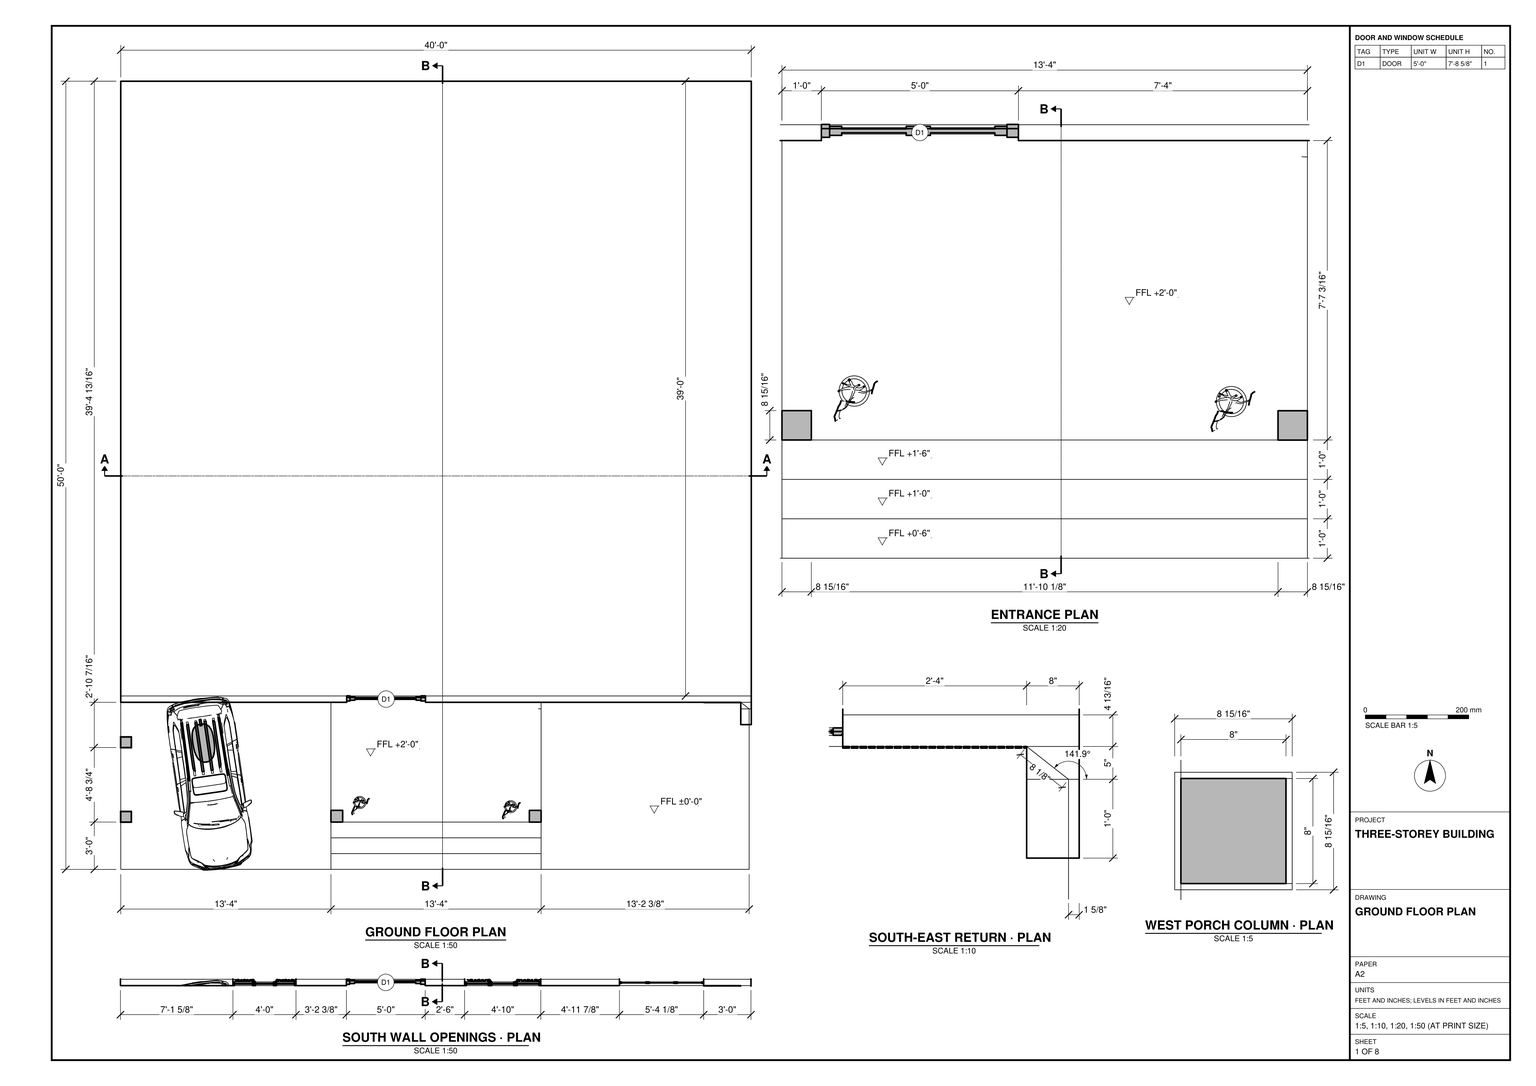
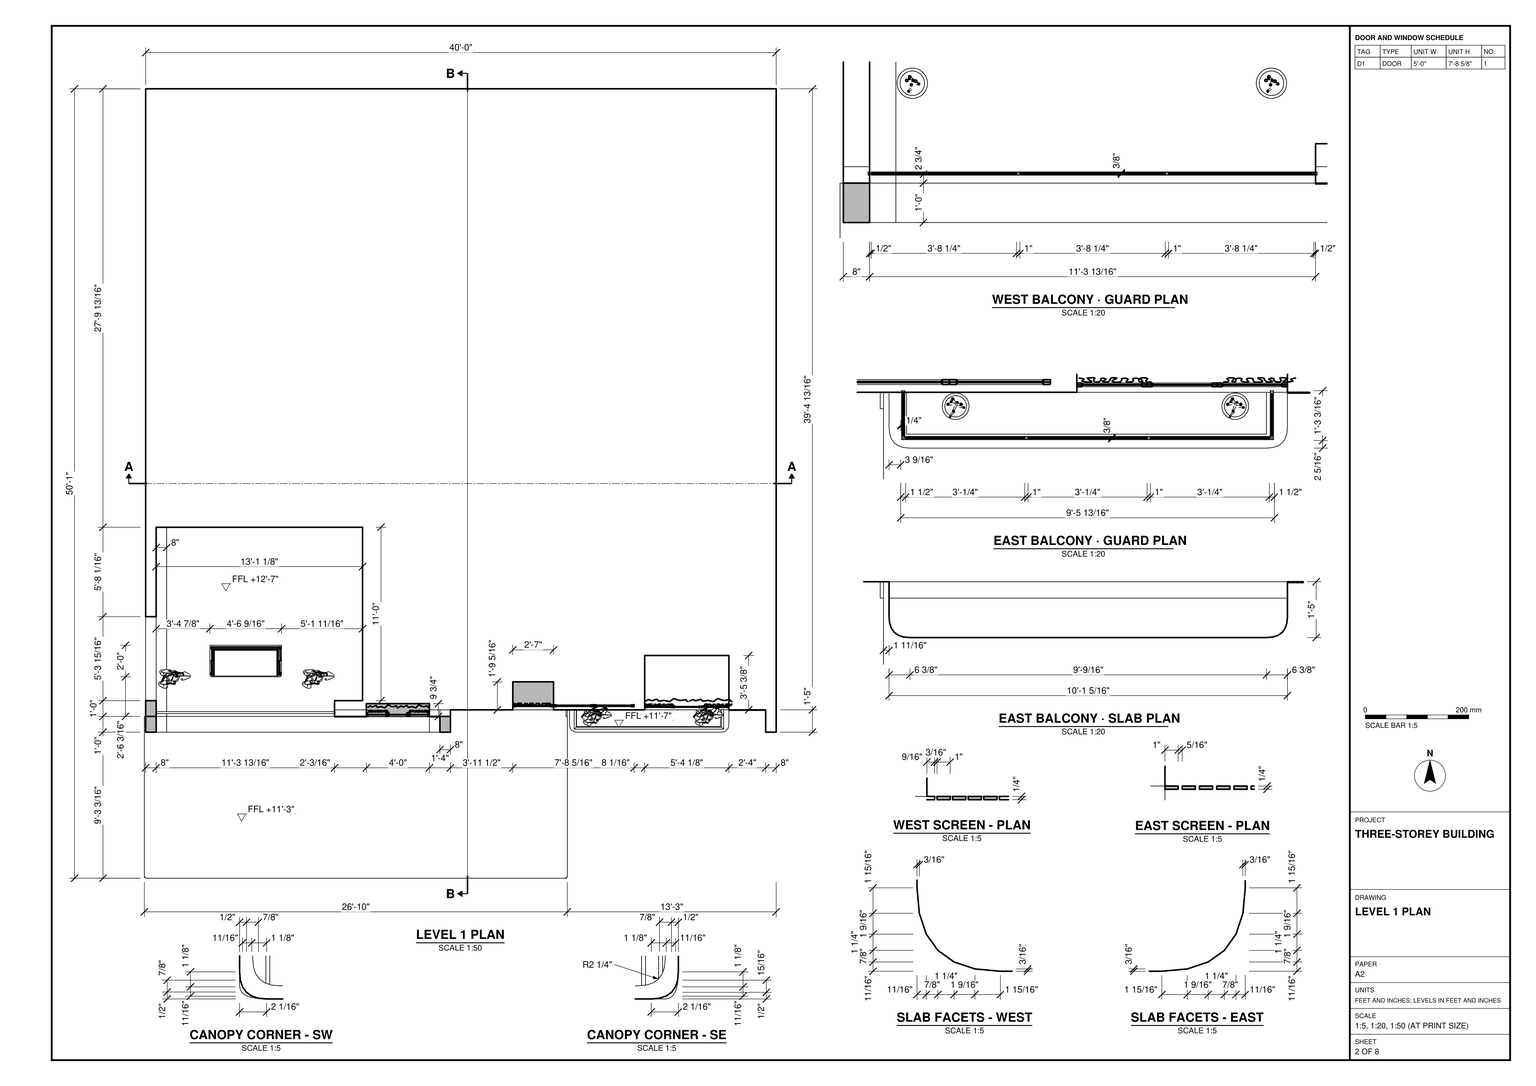
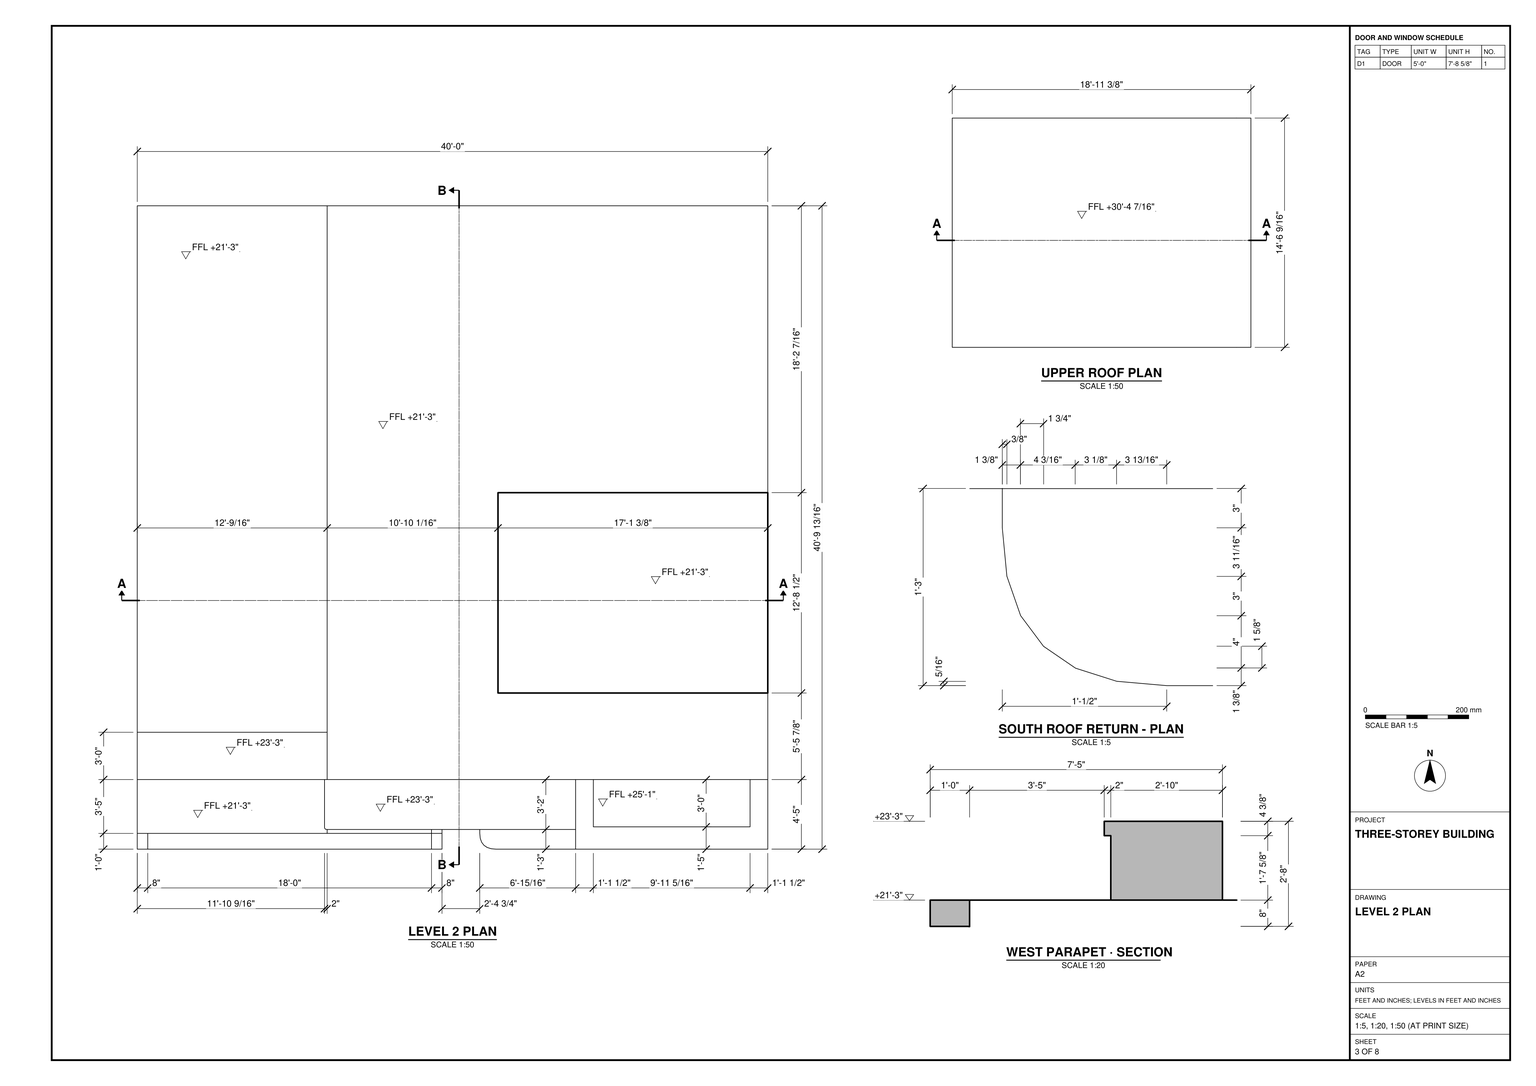
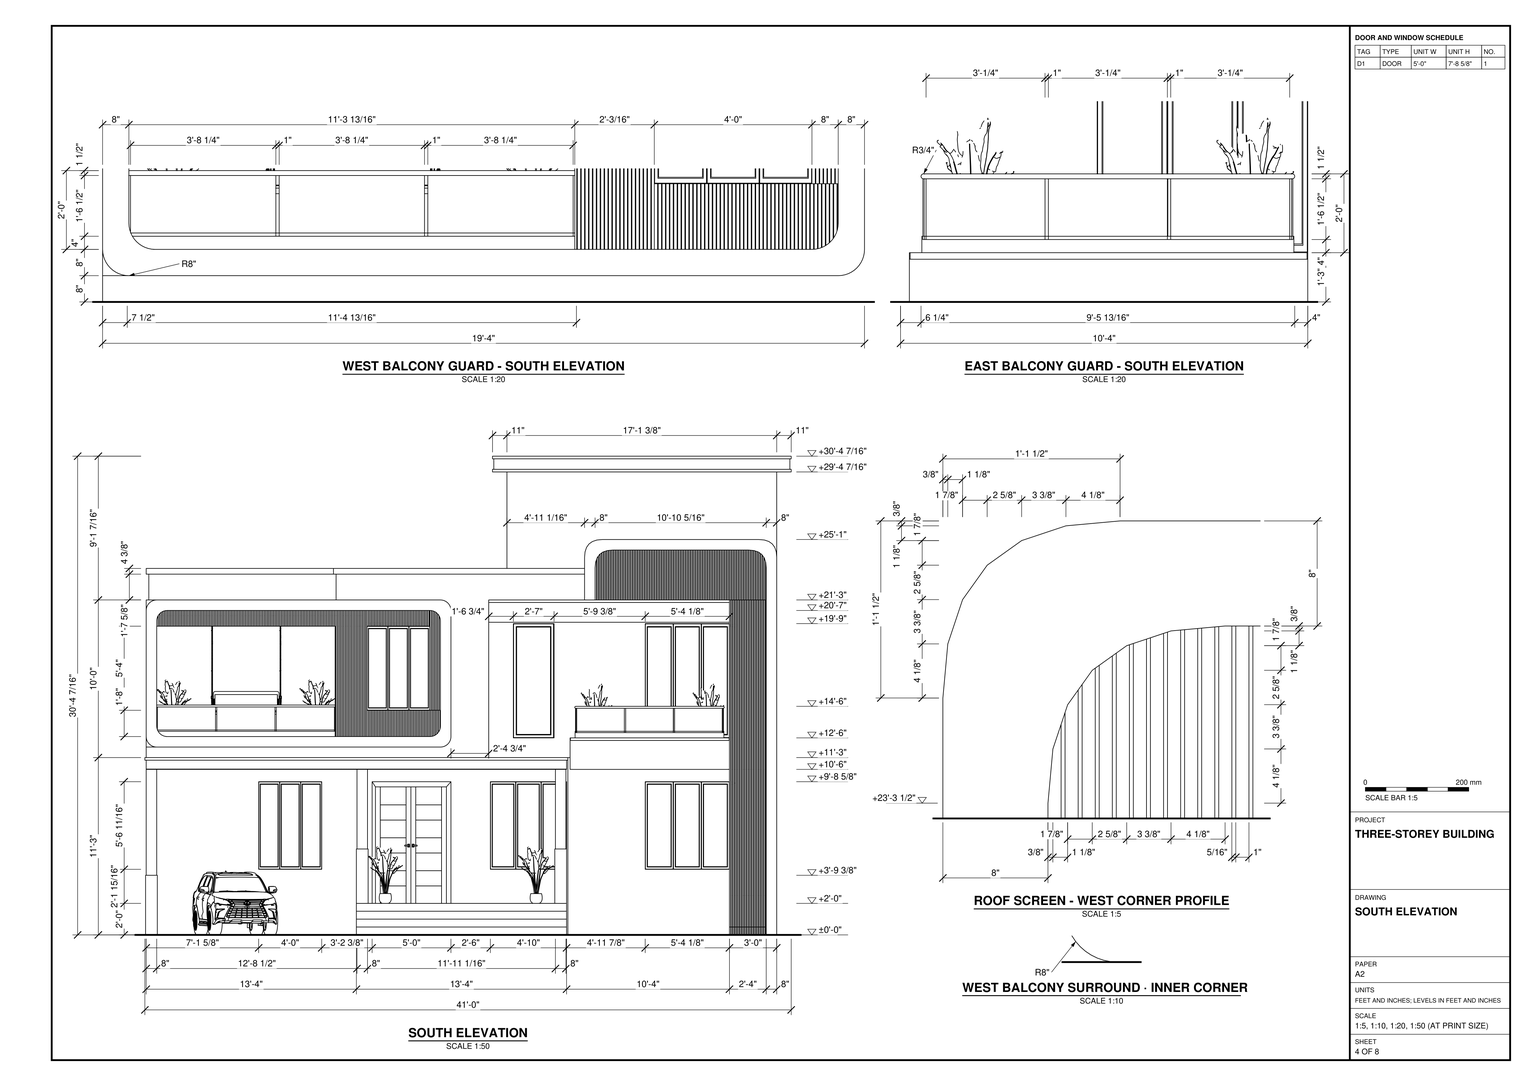
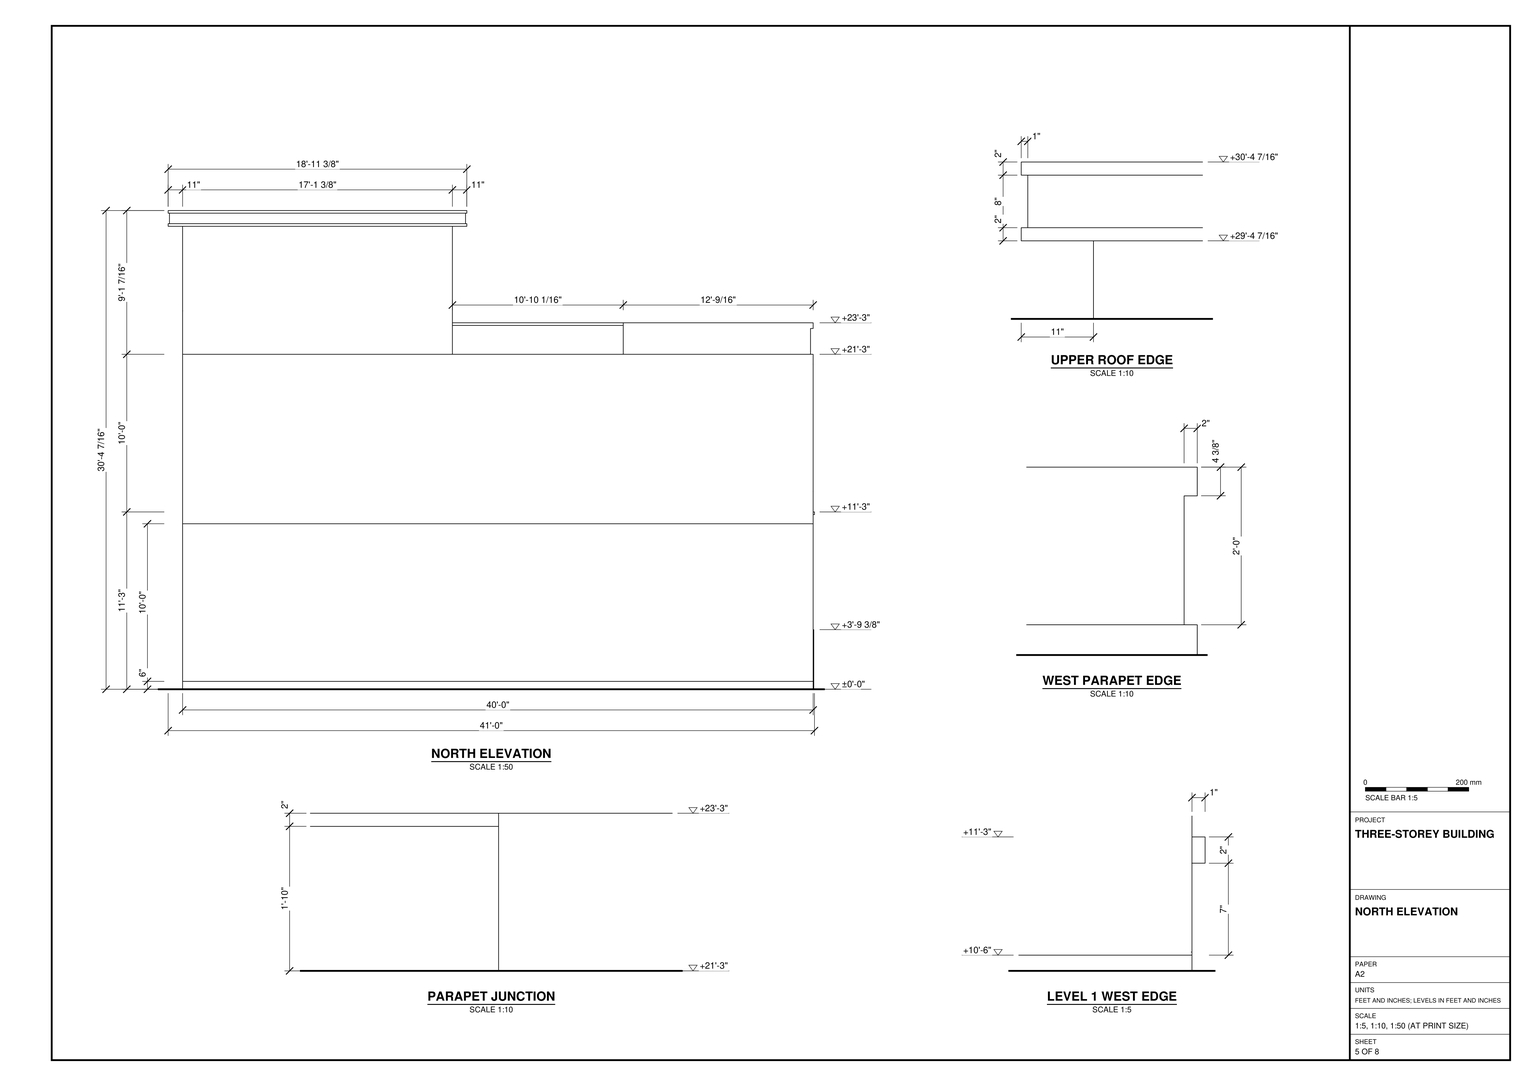
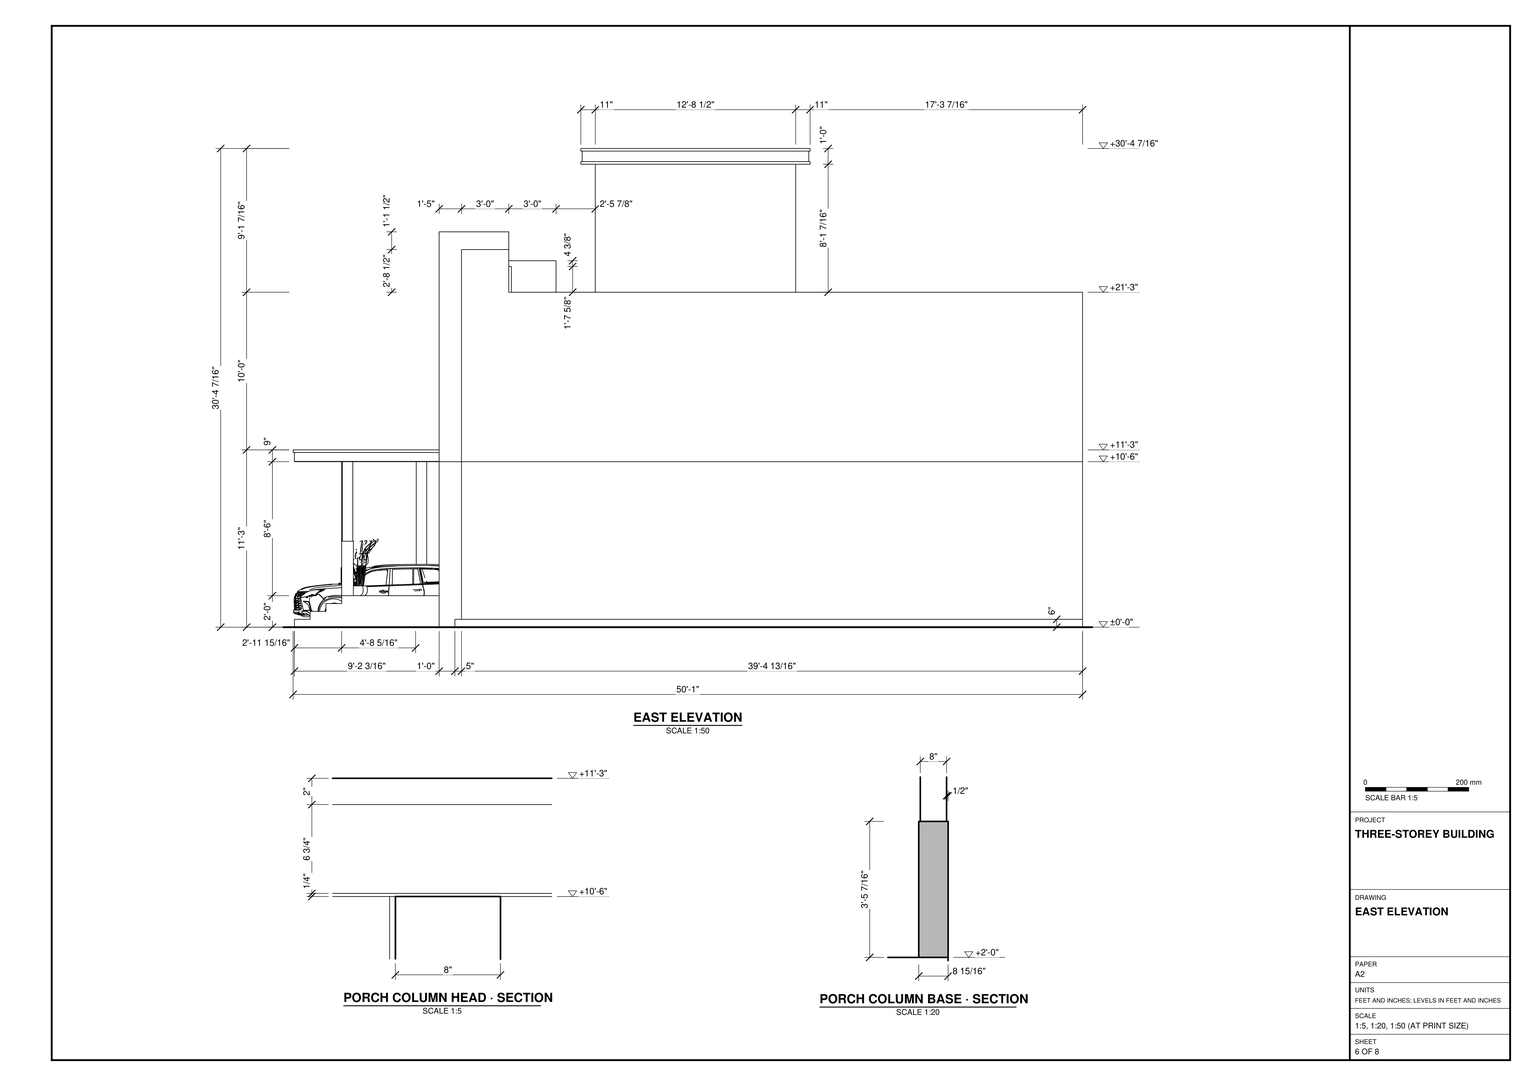
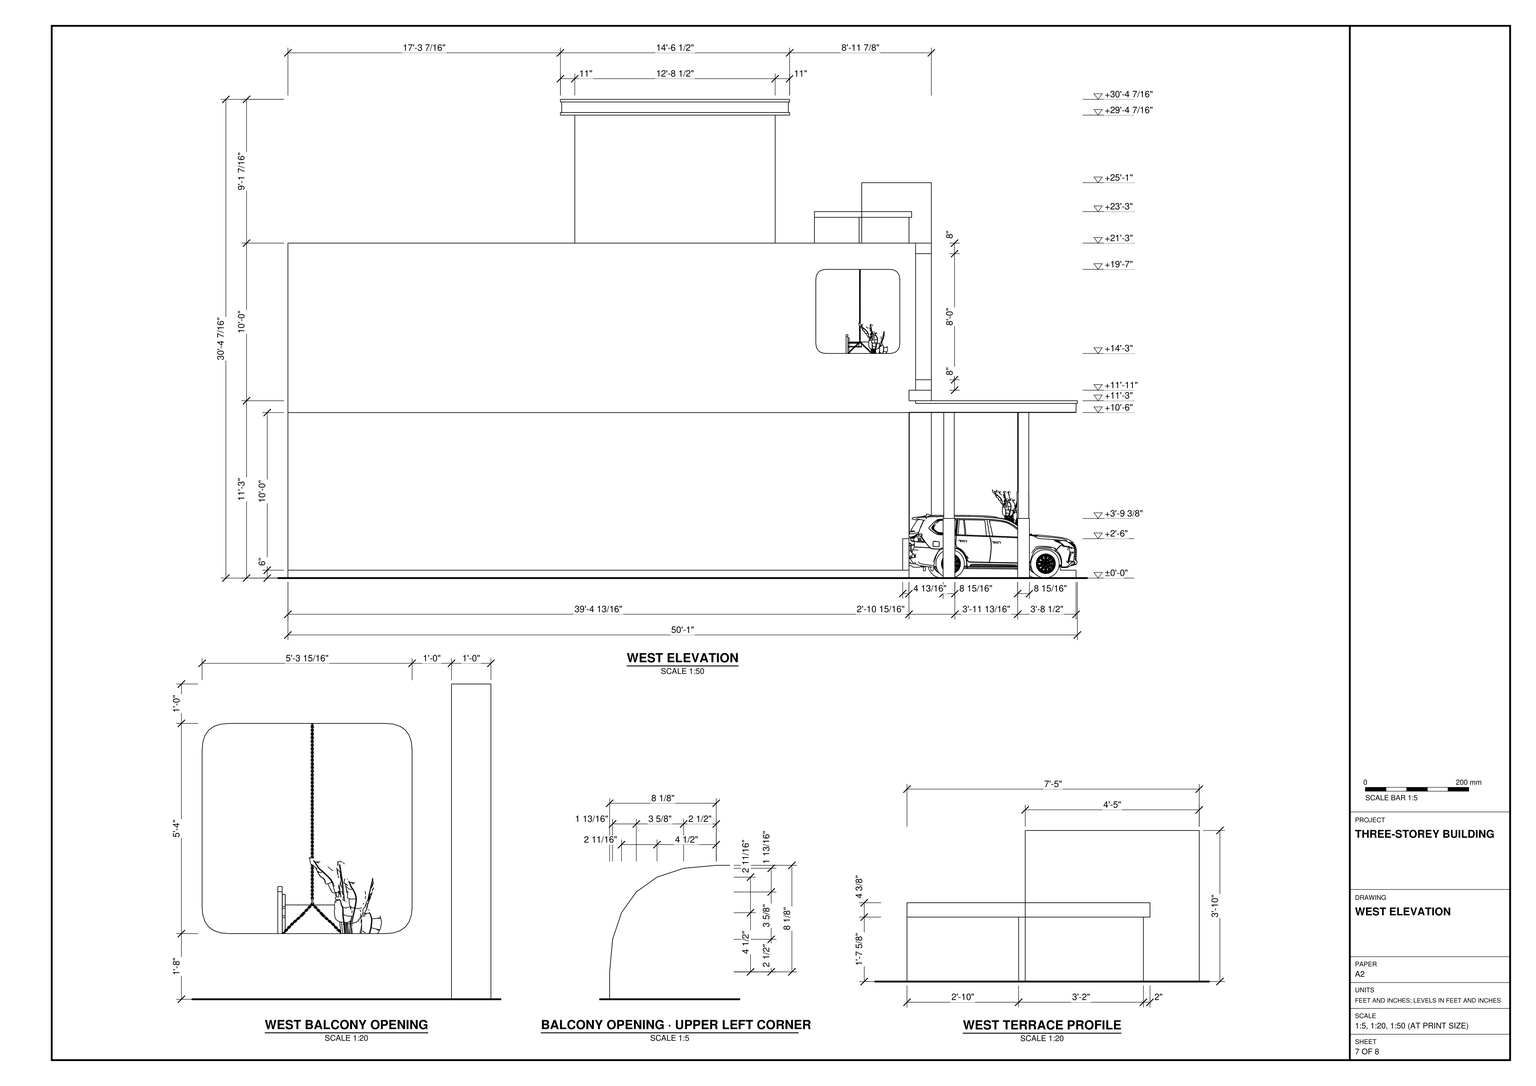
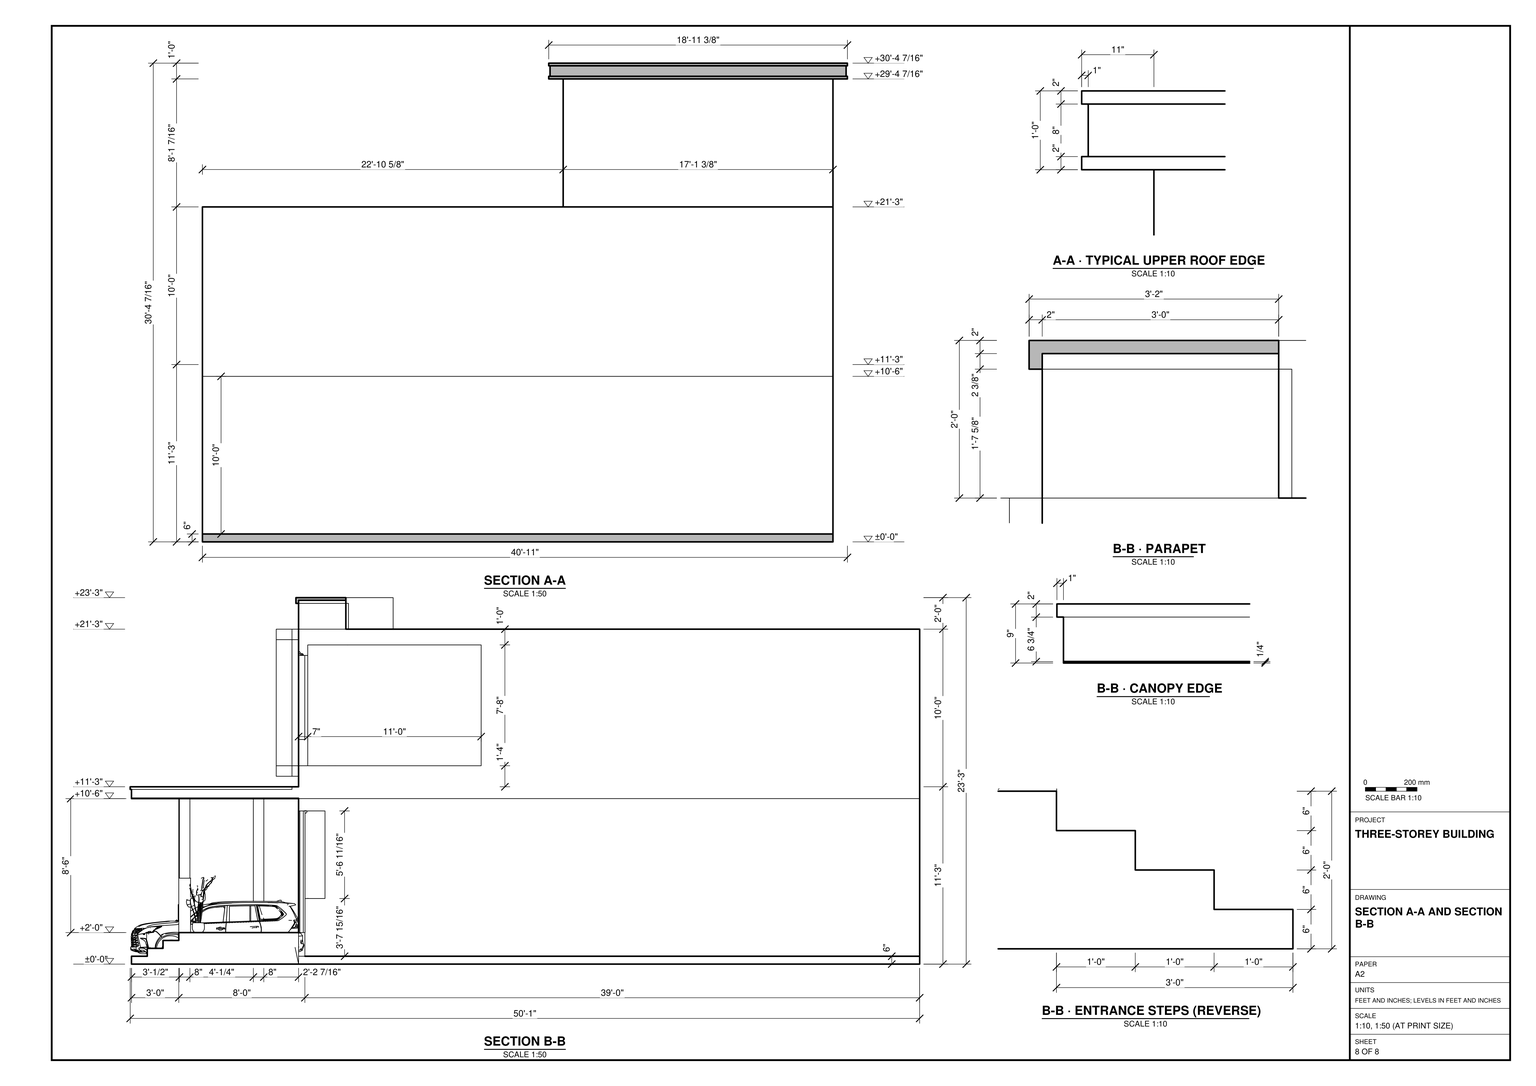
Build the three-storey building in SketchUp from task_files/diagram_01.pdf. Work in feet and inches. The overall model measures 41'-0" along X, 50'-1" along Y and 30'-4 7/16" along Z. Set the ground floor at ±0'-0", Level 1 at +11'-3" and Level 2 at +21'-3". Use the local levels on the sheets for the entrance landing, balconies and parapets.

Lay out the south frontage with the parking bay on the west and the stepped entrance in the middle bay. Carry the steps across the landing frontage and place the double door at the offset shown in the entrance plan. Model the walls at their drawn thicknesses, including the south-east return, and follow the south wall opening layout. Form the floor slabs and the canopy over the parking bay and entrance. Distinguish the recessed west balcony with its straight glass guard from the shallow projecting east balcony with its rounded slab corners and returning guard. Include the screens, parapets, smaller upper enclosure and flat upper roof. Place the vehicle, built-in joinery and main furniture where shown. Decor and loose items may be any suitable library components.

Keep walls, slabs, roof and each furniture or joinery piece in separate groups or components, and use components for repeated parts. Save one SketchUp model as output_files/three_storey_building_with_entrance_steps_and_balconies.skp.

# SketchUp Ruby script. Lengths in inches.
U = 1.inch
M = Sketchup.active_model
def pt(a) = Geom::Point3d.new(a.map { |v| v * U })
def face(e, loops, mat)
  f = e.add_face(loops[0].map { |a| pt(a) })
  loops[1..].each { |l| e.add_face(l.map { |a| pt(a) }).erase! }
  f.material = f.back_material = mat if mat
  f
end
# faces: each face lists its corners as indices into pts; further lists are holes
def faces(e, pts, list, mat = nil) = list.each { |f| face(e, (f[0].is_a?(Array) ? f : [f]).map { |l| l.map { |i| pts[i] } }, mat) }
# xy, xz, yz: faces in a plane at the given z, y or x. An outline is a flat list of corners, or four numbers for a rectangle; further outlines are holes
def ring(l) = l.size == 4 ? [[l[0], l[1]], [l[2], l[1]], [l[2], l[3]], [l[0], l[3]]] : l.each_slice(2).to_a
def flat(e, list, mat, &to3) = list.each { |f| face(e, (f[0].is_a?(Array) ? f : [f]).map { |l| ring(l).map { |u, v| to3.(u, v) } }, mat) }
def xy(e, z, list, mat = nil) = flat(e, list, mat) { |x, y| [x, y, z] }
def xz(e, y, list, mat = nil) = flat(e, list, mat) { |x, z| [x, y, z] }
def yz(e, x, list, mat = nil) = flat(e, list, mat) { |y, z| [x, y, z] }
def lines(e, pts, list) = list.each { |a, b| e.add_line(pt(pts[a]), pt(pts[b])) }
# prism: a flat outline (further loops are holes) pulled along v
def prism(e, loops, v, mat = nil)
  f = face(e, loops, mat); d = Geom::Vector3d.new(v.map { |x| x * U })
  f.pushpull(f.normal.samedirection?(d) ? d.length : -d.length)
end
def box(e, o, s, mat = nil) = prism(e, [[o, [o[0] + s[0], o[1], o[2]], [o[0] + s[0], o[1] + s[1], o[2]], [o[0], o[1] + s[1], o[2]]]], [0, 0, s[2]], mat)
def at(x, y, z, deg = 0) = Geom::Transformation.translation(pt([x, y, z])) * Geom::Transformation.rotation(ORIGIN, Z_AXIS, deg.degrees)
def axes(o, x, y, z) = Geom::Transformation.new([*x, 0, *y, 0, *z, 0, *pt(o).to_a, 1])
def part(name) = M.definitions.add(name)
# library, detail: a bought-in or finely detailed component or shape, given as its bounding box
def library(name, o, s) = part(name).tap { |d| box(d.entities, o, s) }
def detail(e, o, s) = box(e.add_group.entities, o, s)
def put(e, d, t, mat = nil) = e.add_instance(d, t).tap { |i| i.material = mat if mat }
def group(e, t, mat = nil) = e.add_group.tap { |g| g.transformation = t; g.material = mat if mat }.entities
root = M.entities
M.materials.add("POT_TEXTURE_1").color = [172, 172, 172]
M.materials.add("[0136_Charcoal]").color = [35, 35, 35]
M.materials.add("soil1").color = [68, 55, 47]
M.materials.add("тюль").color = [255, 255, 255]
c1 = part("Group\#61")
p = [[0,1.89,0.38],[0,1.89,1.61],[0,0.72,0],[0,0,0.99],[0,0.72,1.99]]
lines(c1.entities,p,[[0,1],[2,0],[3,2],[4,3],[1,4]])
c2 = part("Pleated curtain panel")
xz(c2.entities,2.13,[[4.6,2.7,5.13,80]])
xz(c2.entities,5.27,[[15.31,2.7,16.125,80]])
yz(c2.entities,16.67,[[3.29,2.7,4.74,80]])
# 1 loose lines left out
p = [[1.66,2.25,2.7],[3.22,1.93,2.7],[3.22,1.93,80],[1.66,2.25,80],[3.53,2.38,2.7],[3.53,2.38,80],
  [9.86,2.02,2.7],[10.31,1.94,2.7],[10.31,1.94,80],[9.86,2.02,80],[11.57,2.08,2.7],[11.57,2.08,80],
  [9.23,2.61,2.7],[9.23,2.61,80],[4.47,2.21,2.7],[4.6,2.13,2.7],[4.6,2.13,80],[4.47,2.21,80],
  [5.13,2.13,2.7],[5.61,2.42,2.7],[5.61,2.42,80],[5.13,2.13,80],[11.91,3.91,2.7],[11.91,3.91,80],
  [13.07,2.39,2.7],[13.2,2.07,2.7],[13.2,2.07,80],[13.07,2.39,80],[13.86,2.05,2.7],[13.86,2.05,80],
  [14.78,2.36,2.7],[14.78,2.36,80],[19.11,2.17,2.7],[19.64,2.13,2.7],[19.64,2.13,80],[19.11,2.17,80],
  [20.05,2.2,80],[20.05,2.2,2.7],[0.73,2.89,2.7],[0.73,2.89,80],[4.17,2.57,2.7],[4.17,2.57,80],
  [6.63,2.37,2.7],[7.21,2.1875,2.7],[7.21,2.1875,80],[6.63,2.37,80],[8.1,2.21,2.7],[8.1,2.21,80],
  [8.6875,3.87,2.7],[8.6875,3.87,80],[18.86,2.29,2.7],[18.86,2.29,80],[16.86,2.42,2.7],[17.27,2.32,2.7],
  [17.27,2.32,80],[16.86,2.42,80],[17.64,2.3,2.7],[17.64,2.3,80],[17.8,2.47,2.7],[17.8,2.47,80],
  [18.73,2.57,2.7],[18.73,2.57,80],[2.85,3.77,2.7],[2.85,3.77,80],[6.16,3.6875,2.7],[6.16,3.6875,80],
  [6.49,2.63,2.7],[6.49,2.63,80],[13.52,3.66,2.7],[13.52,3.66,80],[15.24,3.3,2.7],[15.24,3.3,80],
  [16.73,2.58,2.7],[16.73,2.58,80],[17.43,3.97,2.7],[17.43,3.97,80],[3.97,3.43,2.7],[3.97,3.43,80],
  [7.51,4.62,2.7],[7.51,4.62,80],[9.28,3.38,2.7],[9.28,3.38,80],[16.67,3.29,2.7],[16.67,3.29,80],
  [18.67,3.61,2.7],[18.67,3.61,80],[0.95,3.36,2.7],[0.95,3.36,80],[14.95,4.9,2.7],[14.95,4.9,80],
  [1.38,4.43,2.7],[1.38,4.43,80],[4.41,5.3125,2.7],[4.41,5.3125,80],[10.52,5.17,2.7],[10.52,5.17,80],
  [19.17,4.87,2.7],[19.17,4.87,80],[6.02,5.06,2.7],[6.02,5.06,80],[13.64,4.74,2.7],[13.64,4.74,80],
  [2.23,5.46,2.7],[2.23,5.46,80],[8.72,5.1,2.7],[8.72,5.1,80],[11.87,5.08,2.7],[11.87,5.08,80],
  [17.03,5.16,2.7],[17.03,5.16,80],[0.95,4.94,2.7],[0.95,4.94,80],[6.82,5.39,2.7],[6.82,5.39,80],
  [13.01,5.35,2.7],[13.01,5.35,80],[16.125,5.27,2.7],[16.67,4.74,2.7],[16.67,4.74,80],[16.125,5.27,80],
  [0,5.49,2.7],[0,5.49,80],[15.31,5.27,2.7],[15.31,5.27,80],[18.65,5.66,2.7],[18.65,5.66,80],
  [9.31,5.76,2.7],[9.31,5.76,80],[10.5,5.58,2.7],[10.5,5.58,80],[17.3,5.61,80],[17.3,5.61,2.7],
  [3.98,5.8,2.7],[3.98,5.8,80]]
faces(c2.entities,p,[[0,1,2,3],[1,4,5,2],[6,7,8,9],[7,10,11,8],[12,6,9,13],[14,15,16,17],[18,19,20,21],[10,22,23,11],
  [24,25,26,27],[25,28,29,26],[28,30,31,29],[32,33,34,35],[36,34,33,37],[38,0,3,39],[40,14,17,41],[42,43,44,45],
  [43,46,47,44],[46,48,49,47],[50,32,35,51],[52,53,54,55],[53,56,57,54],[56,58,59,57],[60,50,51,61],[4,62,63,5],
  [19,64,65,20],[66,42,45,67],[68,24,27,69],[30,70,71,31],[72,52,55,73],[58,74,75,59],[76,40,41,77],[78,66,67,79],
  [80,12,13,81],[82,72,73,83],[84,60,61,85],[86,38,39,87],[70,88,89,71],[90,86,87,91],[92,76,77,93],[94,80,81,95],
  [96,84,85,97],[64,98,99,65],[100,68,69,101],[62,102,103,63],[48,104,105,49],[22,106,107,23],[74,108,109,75],[110,90,91,111],
  [112,78,79,113],[114,100,101,115],[116,117,118,119],[120,110,111,121],[88,122,123,89],[124,96,97,125],[98,112,113,99],[104,126,127,105],
  [106,114,115,107],[128,94,95,129],[130,109,108,131],[132,92,93,133],[102,132,133,103],[126,128,129,127],[131,124,125,130]])
put(c2.entities,c1,at(9.77,5.02,80,-180))
put(c2.entities,c1,at(11.91,5.02,80,-180))
put(c2.entities,c1,at(13.54,5.02,80,-180))
put(c2.entities,c1,at(7.29,5.02,80,-180))
put(c2.entities,c1,at(6.18,5.02,80,-180))
put(c2.entities,c1,at(8.69,5.02,80,-180))
put(c2.entities,c1,at(17.42,5.04,80,-180))
put(c2.entities,c1,at(18.86,5.04,80,-180))
put(c2.entities,c1,at(15.09,5.02,80,-180))
put(c2.entities,c1,at(16.66,5.04,80,-180))
put(c2.entities,c1,at(2.54,5.02,80,-180))
put(c2.entities,c1,at(1.38,5.02,80,-180))
put(c2.entities,c1,at(4.1,5.02,80,-180))
c3 = part("end")
yz(c3.entities,0,[[1.28,1.02,0.97,1.12,0.97,1.45,1.28,1.55,1.48,1.28]])
p = [[2,0,0.49],[0,0.97,1.12],[0,1.28,1.02],[2,1.51,0],[4,0.54,0.84],[4,1.38,0.57],
  [0,1.48,1.28],[2,2.44,1.28],[4,1.9,1.28],[2,0,2.08],[0,0.97,1.45],[4,0.54,1.72],
  [0,1.28,1.55],[2,1.51,2.57],[4,1.38,2]]
faces(c3.entities,p,[[0,1,2,3],[4,0,3,5],[3,2,6,7],[3,7,8,5],[0,9,10,1],[4,11,9,0],[6,12,13,7],[7,13,14,8],
  [13,12,10,9],[14,13,9,11]])
c4 = part("Component\#75")
p = [[0,2.02,1.1875],[0,1.01,1.92],[0,1.64,0],[0,0,1.1875],[0,0.39,0]]
lines(c4.entities,p,[[0,1],[2,0],[3,4],[4,2],[1,3]])
c5 = part("Shower curtain\#1")
xy(c5.entities,-0.5,[[27.83,-0.5,97.78,0]],"[0136_Charcoal]")
xy(c5.entities,0,[[27.83,-0.5,97.78,0]],"[0136_Charcoal]")
xz(c5.entities,-0.5,[[27.83,-0.5,97.78,0]],"[0136_Charcoal]")
xz(c5.entities,0,[[27.83,-0.5,97.78,0]],"[0136_Charcoal]")
yz(c5.entities,27.83,[[-0.5,-0.5,0,0]])
yz(c5.entities,97.78,[[-0.5,-0.5,0,0]],"[0136_Charcoal]")
put(c5.entities,c4,at(16.28,-1.32,-1.6875))
put(c5.entities,c4,at(12.125,-1.32,-1.6875))
put(c5.entities,c4,at(25.09,-1.32,-1.6875))
put(c5.entities,c4,at(7.66,-1.32,-1.6875))
put(c5.entities,c4,at(37.05,-1.32,-1.6875))
put(c5.entities,c4,at(48.17,-1.32,-1.6875))
put(c5.entities,c4,at(29.99,-1.32,-1.6875))
put(c5.entities,c4,at(34.45,-1.32,-1.6875))
put(c5.entities,c4,at(58.19,-1.32,-1.6875))
put(c5.entities,c4,at(52.32,-1.32,-1.6875))
put(c5.entities,c4,at(3.19,-1.32,-1.6875))
put(c5.entities,c4,at(21.06,-1.32,-1.6875))
put(c5.entities,c4,at(43.39,-1.32,-1.6875))
g1 = group(c5.entities,at(0.71,-1.3,-104.16))
p = [[26.9375,4.31,0],[20.6,5.3,0.1],[20.6,0.99,102.68],[26.9375,0,102.58],[31.63,6.62,0.24],[31.63,2.31,102.82],
  [47.72,4.31,0],[46.34,4.86,0.06],[46.34,0.55,102.64],[47.72,0,102.58],[14.89,4.64,0.03],[12.6875,6.18,0.19],
  [12.6875,1.87,102.77],[14.89,0.33,102.61],[3.59,5.85,0.16],[0,4.86,0.06],[0,0.55,102.64],[3.59,1.54,102.74],
  [45.42,5.85,0.16],[45.42,1.54,102.74],[6.9,4.97,0.07],[6.9,0.66,102.65],[39.72,5.1875,0.09],[35.58,5.625,0.14],
  [35.58,1.32,102.72],[39.72,0.88,102.67],[34.85,6.07,0.18],[34.85,1.76,102.76]]
faces(g1,p,[[0,1,2,3],[4,0,3,5],[6,7,8,9],[10,11,12,13],[1,10,13,2],[14,15,16,17],[7,18,19,8],[20,14,17,21],
  [11,20,21,12],[22,23,24,25],[18,22,25,19],[23,26,27,24],[26,4,5,27]],"тюль")
g2 = group(c5.entities,at(50.2,-1.3,-104.16))
p = [[26.9375,4.31,0],[20.6,5.3,0.1],[20.6,0.99,102.68],[26.9375,0,102.58],[31.63,6.62,0.24],[31.63,2.31,102.82],
  [47.72,4.31,0],[46.34,4.86,0.06],[46.34,0.55,102.64],[47.72,0,102.58],[14.89,4.64,0.03],[12.6875,6.18,0.19],
  [12.6875,1.87,102.77],[14.89,0.33,102.61],[3.59,5.85,0.16],[0,4.86,0.06],[0,0.55,102.64],[3.59,1.54,102.74],
  [45.42,5.85,0.16],[45.42,1.54,102.74],[6.9,4.97,0.07],[6.9,0.66,102.65],[39.72,5.1875,0.09],[35.58,5.625,0.14],
  [35.58,1.32,102.72],[39.72,0.88,102.67],[34.85,6.07,0.18],[34.85,1.76,102.76]]
faces(g2,p,[[0,1,2,3],[4,0,3,5],[6,7,8,9],[10,11,12,13],[1,10,13,2],[14,15,16,17],[7,18,19,8],[20,14,17,21],
  [11,20,21,12],[22,23,24,25],[18,22,25,19],[23,26,27,24],[26,4,5,27]],"тюль")
c6 = part("Группа\#112")
xy(c6.entities,1.36,[[27.84,0.35,98.7,1.5]],"[0136_Charcoal]")
p = [[98.7,0.92,0],[98.7,0,0.52],[27.84,0,0.52],[27.84,0.92,0],[98.7,1.85,0.52],[27.84,1.85,0.52],
  [98.7,0.35,1.36],[27.84,0.35,1.36],[98.7,1.5,1.36],[27.84,1.5,1.36]]
faces(c6.entities,p,[[0,1,2,3],[4,0,3,5],[1,6,7,2],[8,4,5,9]],"[0136_Charcoal]")
c7 = part("шторы раздвинутые\#1")
put(c7.entities,c2,axes([27.83,-81.89,6.88],[1,0,0],[0,0,-0.36],[0,1,0]))
put(c7.entities,c2,axes([88.28,-81.89,6.88],[-1,0,0],[0,0,-0.36],[0,1,0]))
put(c7.entities,c3,axes([23.6875,-2.09,5.41],[1,0,0],[0,0,-1],[0,1,0]),"[0136_Charcoal]")
put(c7.entities,c3,axes([92,-2.09,5.41],[-1,0,0],[0,0,-1],[0,1,0]),"[0136_Charcoal]")
put(c7.entities,c5,axes([27.39,-1.5,1.72],[0.62018,0,0],[0,-0.03238,-0.99912],[0,0.7459,-0.04059]))
put(c7.entities,c6,axes([4,-1.52,3.51],[0.85105,0,0],[0,0.77173,0],[0,0,1]))
c8 = library("Group\#94",[-662.41,217.3,320.04],[397.32,658.3,1732.06])
c9 = library("Group\#96",[-299.2,181.55,262.58],[360.65,735.71,1258.34])
c10 = library("Group\#91",[-1038.76,656.55,345.34],[733.18,460.51,2065.7])
c11 = library("Group\#89",[-445.29,890.31,329.28],[284.3,304.08,2023.29])
c12 = library("Group\#92",[-733.48,439.625,202.64],[456.28,533.12,1536.78])
c13 = library("Group\#95",[-455.56,899.32,410.78],[341.21,610.33,1581.5])
c14 = library("Group\#88",[-516.34,626.77,-4.5625],[517.73,515.95,418.98])
c15 = library("Group\#93",[-249.24,914.85,310.18],[345.55,647.95,1307.93])
c16 = library("Group\#90",[-277.97,488.68,287.26],[362.84,405.94,1768.54])
c17 = library("Group\#87",[-468.76,669.89,380.1875],[424.36,427.47,41.99])
c18 = part("Potted plant")
put(c18.entities,c8,at(1038.76,-181.55,4.5625))
put(c18.entities,c9,at(1038.76,-181.55,4.5625))
put(c18.entities,c10,at(1038.76,-181.55,4.5625))
put(c18.entities,c11,at(1038.76,-181.55,4.5625))
put(c18.entities,c12,at(1038.76,-181.55,4.5625))
put(c18.entities,c13,at(1038.76,-181.55,4.5625))
put(c18.entities,c14,at(1038.76,-181.55,4.5625),"POT_TEXTURE_1")
put(c18.entities,c15,at(1038.76,-181.55,4.5625))
put(c18.entities,c16,at(1038.76,-181.55,4.5625))
put(c18.entities,c17,at(1038.76,-181.55,4.5625),"soil1")
c19 = part("plants(2)")
put(c19.entities,c18,axes([-3298.7,16879.33,962.02],[0.26233,-0.53859,0],[0.53859,0.26233,0],[0,0,0.59908]))
put(c19.entities,c18,axes([-7168.4,16988.26,962.02],[0.26361,-0.54122,0],[0.54122,0.26361,0],[0,0,0.602]))
put(c19.entities,c18,axes([-1678.07,19377.75,4834.08],[0.22822,-0.46857,0],[0.47934,0.23347,0],[0,0,0.74285]))
put(c19.entities,c18,axes([1189.32,19377.75,4834.08],[0.22822,-0.46857,0],[0.47934,0.23347,0],[0,0,0.74285]))
put(c19.entities,c18,axes([-8907.24,20412.17,5238.12],[0.26361,-0.54122,0],[0.54122,0.26361,0],[0,0,0.602]))
put(c19.entities,c18,axes([-12589.9,20412.17,5238.12],[0.26361,-0.54122,0],[0.54122,0.26361,0],[0,0,0.602]))
c20 = library("sWING-1250",[0,0,16],[54.55,24,105.18])
c21 = library("Group\#1",[-1,-4.35,0],[492,604.35,364.4375])
put(root,c7,axes([266.45,10.96,236.46],[1.09,0,0],[0,0,1.08938],[0,-1,0]))
put(root,c7,axes([268.77,15.35,116.23],[1.03745,0,0],[0,0,0.83522],[0,-1,0]))
put(root,c7,axes([154.68,11.18,116.61],[0.9156,0,0],[0,0,0.84006],[0,-1,0]))
put(root,c7,axes([-18.15,11.18,116.61],[0.76595,0,0],[0,0,0.84006],[0,-1,0]))
put(root,c7,axes([64.23,6.18,237.67],[0.76595,0,0],[0,0,0.84006],[0,-1,0]))
put(root,c19,axes([293.7,-572.07,-4.57],[0.0297,0,0],[0,0.0297,0],[0,0,0.0297]))
put(root,c20,axes([-34.92,26.89,156.55],[1,0,0],[0,1,0],[0,0,0.7134]))
put(root,c21,at(-83.79,-125.48,0))
